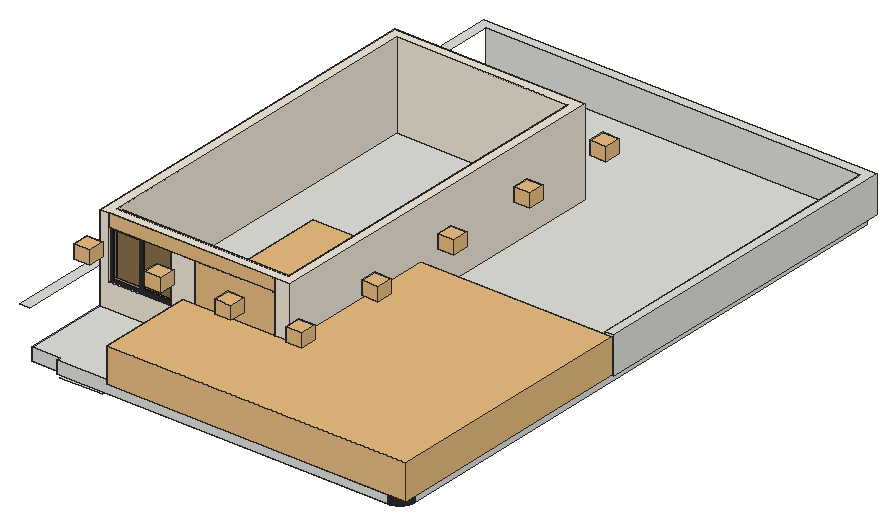
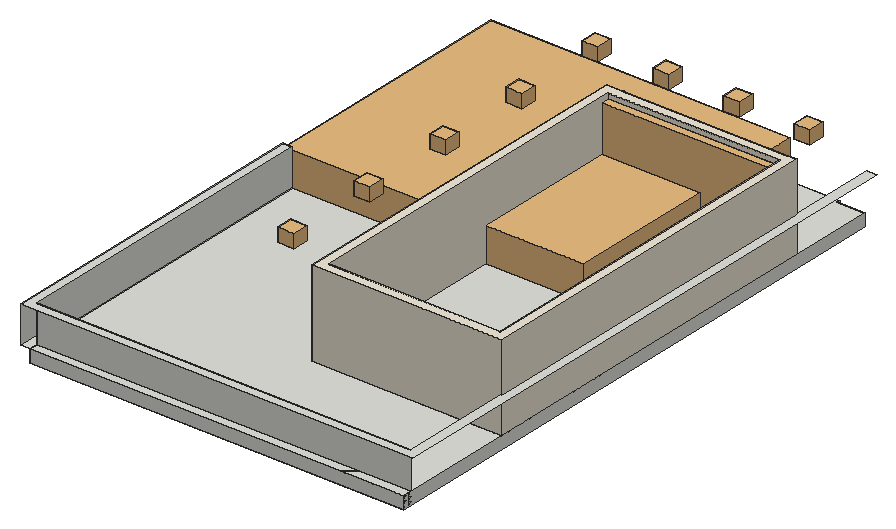
# SketchUp Ruby script. Lengths in inches.
U = 1.inch
M = Sketchup.active_model
def pt(a) = Geom::Point3d.new(a.map { |v| v * U })
def face(e, loops, mat)
  f = e.add_face(loops[0].map { |a| pt(a) })
  loops[1..].each { |l| e.add_face(l.map { |a| pt(a) }).erase! }
  f.material = f.back_material = mat if mat
  f
end
# faces: each face lists its corners as indices into pts; further lists are holes
def faces(e, pts, list, mat = nil) = list.each { |f| face(e, (f[0].is_a?(Array) ? f : [f]).map { |l| l.map { |i| pts[i] } }, mat) }
# xy, xz, yz: faces in a plane at the given z, y or x. An outline is a flat list of corners, or four numbers for a rectangle; further outlines are holes
def ring(l) = l.size == 4 ? [[l[0], l[1]], [l[2], l[1]], [l[2], l[3]], [l[0], l[3]]] : l.each_slice(2).to_a
def flat(e, list, mat, &to3) = list.each { |f| face(e, (f[0].is_a?(Array) ? f : [f]).map { |l| ring(l).map { |u, v| to3.(u, v) } }, mat) }
def xy(e, z, list, mat = nil) = flat(e, list, mat) { |x, y| [x, y, z] }
def xz(e, y, list, mat = nil) = flat(e, list, mat) { |x, z| [x, y, z] }
def yz(e, x, list, mat = nil) = flat(e, list, mat) { |y, z| [x, y, z] }
def lines(e, pts, list) = list.each { |a, b| e.add_line(pt(pts[a]), pt(pts[b])) }
# prism: a flat outline (further loops are holes) pulled along v
def prism(e, loops, v, mat = nil)
  f = face(e, loops, mat); d = Geom::Vector3d.new(v.map { |x| x * U })
  f.pushpull(f.normal.samedirection?(d) ? d.length : -d.length)
end
def box(e, o, s, mat = nil) = prism(e, [[o, [o[0] + s[0], o[1], o[2]], [o[0] + s[0], o[1] + s[1], o[2]], [o[0], o[1] + s[1], o[2]]]], [0, 0, s[2]], mat)
def at(x, y, z, deg = 0) = Geom::Transformation.translation(pt([x, y, z])) * Geom::Transformation.rotation(ORIGIN, Z_AXIS, deg.degrees)
def axes(o, x, y, z) = Geom::Transformation.new([*x, 0, *y, 0, *z, 0, *pt(o).to_a, 1])
def part(name) = M.definitions.add(name)
# library, detail: a bought-in or finely detailed component or shape, given as its bounding box
def library(name, o, s) = part(name).tap { |d| box(d.entities, o, s) }
def detail(e, o, s) = box(e.add_group.entities, o, s)
def put(e, d, t, mat = nil) = e.add_instance(d, t).tap { |i| i.material = mat if mat }
def group(e, t, mat = nil) = e.add_group.tap { |g| g.transformation = t; g.material = mat if mat }.entities
root = M.entities
M.materials.add("0027 AP L140 CRUSHED ICE").color = [241, 233, 217]
M.materials.add("Glass_Tinted_Gray").color = [0, 0, 0]
M.materials["Glass_Tinted_Gray"].alpha = 0.125
M.materials.add("[0135_DarkGray]").color = [81, 81, 81]
M.materials.add("[Metal Seamed]").color = [40, 40, 40]
M.materials.add("[Mirror 02]").color = [229, 229, 229]
M.materials.add("[Terrazzo Light Blue]").color = [196, 214, 227]
M.materials.add("[Wood Cherry Original]").color = [103, 58, 28]
M.materials.add("[Wood Fence]").color = [142, 67, 30]
c1 = library("Sliding glass door",[0,0,0],[5.83,106.3,82.68])
c2 = library("Group\#37",[0,0,0],[292,251.5,34])
c3 = library("Curtains",[0,0,0],[121.73,8.19,117.22])
c4 = library("Group\#52",[0,-0.5,0],[162,0.5,12])
c5 = part("PENTEK_RP Fineline 50S_Sliding_DoorCase_E1")
box(c5.entities,[0,0,0],[1.51,3.66,99.27],"[0135_DarkGray]")
c6 = part("PENTEK_RP Fineline 50S_SlidingDooe_Case_E2")
box(c6.entities,[0,0,0],[96.25,3.66,1.51],"[0135_DarkGray]")
c7 = part("pentek_RP Fineline 50S_SlidingDoor_Case")
put(c7.entities,c5,at(97.76,0,0))
put(c7.entities,c6,at(1.51,0,0))
put(c7.entities,c5,at(0,0,0))
put(c7.entities,c6,at(1.51,0,97.76))
c8 = part("PENTEK_RP Fineline 50S_SlidingDoor_GlazingBead_2")
box(c8.entities,[0,0,0],[0.56,0.59,94.39],"[0135_DarkGray]")
c9 = part("PENTEK_RP Fineline 50S_SlidingDoor_Glass")
box(c9.entities,[0,0,0],[46.58,0.16,94.39],"Glass_Tinted_Gray")
c10 = part("PENTEK_RP Fineline 50S_SlidingDoor_GlazingBead")
box(c10.entities,[0,0,0],[45.47,0.59,0.56],"[0135_DarkGray]")
c11 = part("PENTEK_RP Fineline 50S_SlidingDoor_Leaf_E1")
xy(c11.entities,0,[[0,0,0.93,1.97],[0.93,1.57,1.49,1.97]],"[0135_DarkGray]")
xy(c11.entities,96.25,[[0,0,0.93,0,0.93,1.57,1.49,1.57,1.49,1.97,0,1.97]],"[0135_DarkGray]")
xz(c11.entities,0,[[0,0,0.93,96.25]],"[0135_DarkGray]")
xz(c11.entities,1.57,[[0.93,0,1.49,95.32],[0.93,95.32,1.49,96.25]],"[0135_DarkGray]")
xz(c11.entities,1.97,[[0,0,1.49,96.25]],"[0135_DarkGray]")
yz(c11.entities,0,[[0,0,1.97,96.25]],"[0135_DarkGray]")
yz(c11.entities,0.93,[[0,0,1.57,0.93],[0,0.93,1.57,95.32],[0,95.32,1.57,96.25]],"[0135_DarkGray]")
yz(c11.entities,1.49,[[1.57,0,1.97,95.32],[1.57,95.32,1.97,96.25]],"[0135_DarkGray]")
c12 = part("PENTEK_RP Fineline 50S_SlidingDoor_Leaf_E2")
xy(c12.entities,0,[[0,0,0,1.57,0.56,1.57,0.56,1.97,46.02,1.97,46.02,1.57,46.58,1.57,46.58,0]],"[0135_DarkGray]")
xy(c12.entities,0.93,[[0,0,46.58,1.57]],"[0135_DarkGray]")
xy(c12.entities,1.49,[[0.56,1.57,46.02,1.97]],"[0135_DarkGray]")
xz(c12.entities,0,[[0,0,46.58,0.93]],"[0135_DarkGray]")
xz(c12.entities,1.57,[[0,0,0.56,0.93],[46.02,0,46.58,0.93],[0.56,0.93,46.02,1.49]],"[0135_DarkGray]")
xz(c12.entities,1.97,[[0.56,0,46.02,1.49]],"[0135_DarkGray]")
yz(c12.entities,0,[[0,0,1.57,0.93]],"[0135_DarkGray]")
yz(c12.entities,0.56,[[1.57,0,1.97,0.93],[1.57,0.93,1.97,1.49]],"[0135_DarkGray]")
yz(c12.entities,46.02,[[1.57,0,1.97,0.93],[1.57,0.93,1.97,1.49]],"[0135_DarkGray]")
yz(c12.entities,46.58,[[0,0,1.57,0.93]],"[0135_DarkGray]")
c13 = part("PENTEK_RP Fineline S_SlidingDoor_Leaf1")
put(c13.entities,c8,at(0.93,0,0.93))
put(c13.entities,c8,at(46.96,0,0.93))
put(c13.entities,c9,at(1.49,1.42,0.93))
put(c13.entities,c10,at(1.49,0,0.93))
put(c13.entities,c9,at(1.49,0.59,0.93),"[Terrazzo Light Blue]")
put(c13.entities,c11,at(0,0,0))
put(c13.entities,c11,axes([48.44,0,0],[-1,0,0],[0,1,0],[0,0,1]))
put(c13.entities,c12,axes([0.93,0,96.25],[1,0,0],[0,1,0],[0,0,-1]))
put(c13.entities,c12,at(0.93,0,0))
put(c13.entities,c10,at(1.49,0,94.77))
c14 = part("PENTEK_RP Fineline 50S_SlidingDoor_Leaf2")
put(c14.entities,c9,at(1.49,1.42,0.93))
put(c14.entities,c10,at(1.49,0,94.77))
put(c14.entities,c8,at(46.96,0,0.93))
put(c14.entities,c9,at(1.49,0.59,0.93),"[Mirror 02]")
put(c14.entities,c8,at(0.93,0,0.93))
put(c14.entities,c11,at(0,0,0))
put(c14.entities,c11,axes([48.44,0,0],[-1,0,0],[0,1,0],[0,0,1]))
put(c14.entities,c10,at(1.49,0,0.93))
put(c14.entities,c12,axes([0.93,0,96.25],[1,0,0],[0,1,0],[0,0,-1]))
put(c14.entities,c12,at(0.93,0,0))
c15 = part("PENTEK - Slimmest Steel Sliding Door / Window\#1")
put(c15.entities,c7,at(0,-1.88,-0.09))
put(c15.entities,c13,at(1.51,-2.27,1.42))
put(c15.entities,c14,at(49.32,-0.3,1.42))
c16 = library("3",[-5.94,-5.94,-13.08],[15.84,15.84,13.08])
xy(root,234,[[55.37,255,55.29,255.01,55.21,255.01,55.13,255.02,55.06,255.03,54.98,255.05,54.9,255.06,54.82,255.08,54.75,255.1,54.67,255.12,54.6,255.14,54.52,255.16,54.45,255.19,54.3,255.25,54.23,255.28,54.16,255.32,54.09,255.35,53.95,255.43,53.89,255.47,53.82,255.51,53.76,255.56,53.69,255.6,53.51,255.75,53.29,255.97,53.24,256.03,53.18,256.09,53.14,256.15,53.09,256.22,53.04,256.28,53,256.34,52.96,256.41,52.91,256.48,52.84,256.62,52.8,256.6875,52.77,256.76,52.68,256.97,52.65,257.05,52.61,257.2,52.59,257.28,52.57,257.35,52.55,257.43,52.54,257.51,52.53,257.58,52.51,257.74,52.51,257.82,52.5,257.9,52.5,258.13,52.51,258.21,52.51,258.29,52.52,258.37,52.53,258.44,52.55,258.52,52.56,258.6,52.58,258.68,52.6,258.75,52.62,258.83,52.64,258.9,52.66,258.98,52.69,259.05,52.75,259.2,52.78,259.27,52.82,259.34,52.85,259.41,52.93,259.55,52.97,259.61,53.01,259.68,53.06,259.74,53.1,259.81,53.25,259.99,53.47,260.21,53.53,260.26,53.59,260.32,53.65,260.36,53.72,260.41,53.78,260.46,53.84,260.5,53.91,260.54,53.98,260.59,54.12,260.66,54.1875,260.7,54.26,260.73,54.47,260.82,54.55,260.85,54.7,260.89,54.78,260.91,54.85,260.93,54.93,260.95,55.01,260.96,55.08,260.97,55.24,260.99,55.32,260.99,55.4,261,55.63,261,55.71,260.99,55.79,260.99,55.87,260.98,55.94,260.97,56.02,260.95,56.1,260.94,56.18,260.92,56.25,260.9,56.33,260.88,56.4,260.86,56.48,260.84,56.55,260.81,56.7,260.75,56.77,260.72,56.84,260.68,56.91,260.65,57.05,260.57,57.11,260.53,57.18,260.49,57.24,260.44,57.31,260.4,57.49,260.25,57.71,260.03,57.76,259.97,57.82,259.91,57.86,259.85,57.91,259.78,57.96,259.72,58,259.66,58.04,259.59,58.09,259.52,58.16,259.38,58.2,259.3125,58.23,259.24,58.32,259.03,58.35,258.95,58.39,258.8,58.41,258.72,58.43,258.65,58.45,258.57,58.46,258.49,58.47,258.42,58.49,258.26,58.49,258.18,58.5,258.1,58.5,257.87,58.49,257.79,58.49,257.71,58.48,257.63,58.47,257.56,58.45,257.48,58.44,257.4,58.42,257.32,58.4,257.25,58.38,257.17,58.36,257.1,58.34,257.02,58.31,256.95,58.25,256.8,58.22,256.73,58.18,256.66,58.15,256.59,58.07,256.45,58.03,256.39,57.99,256.32,57.94,256.26,57.9,256.19,57.75,256.01,57.53,255.79,57.47,255.74,57.41,255.68,57.35,255.64,57.28,255.59,57.22,255.54,57.16,255.5,57.09,255.46,57.02,255.41,56.88,255.34,56.8125,255.3,56.74,255.27,56.53,255.18,56.45,255.15,56.3,255.11,56.22,255.09,56.15,255.07,56.07,255.05,55.99,255.04,55.92,255.03,55.76,255.01,55.68,255.01,55.6,255]],"[Wood Fence]")
xy(root,252,[[51,210,93,210,93,213,99,213,99,214,368.95,214,369.1,214.01,369.29,214.04,369.48,214.0625,369.67,214.09,369.85,214.12,370.23,214.18,370.42,214.22,370.61,214.25,370.8,214.29,370.98,214.34,371.17,214.38,371.35,214.43,371.54,214.48,371.72,214.53,371.91,214.58,372.45,214.76,372.64,214.82,372.82,214.89,372.99,214.95,373.17,215.02,373.35,215.1,373.53,215.17,373.7,215.25,373.88,215.32,374.05,215.41,374.22,215.49,374.4,215.57,374.91,215.84,375.07,215.93,375.24,216.03,375.4,216.125,375.57,216.22,375.73,216.32,375.89,216.43,376.05,216.53,376.37,216.75,376.52,216.86,376.68,216.97,376.83,217.09,376.98,217.2,377.43,217.56,377.58,217.6875,377.72,217.8125,377.86,217.94,378.01,218.07,378.15,218.2,378.56,218.61,378.6875,218.74,378.82,218.88,378.95,219.02,379.08,219.17,379.2,219.31,379.33,219.46,379.45,219.6,379.81,220.05,379.92,220.21,380.04,220.36,380.15,220.52,380.26,220.67,380.36,220.83,380.47,220.99,380.57,221.15,380.68,221.31,380.78,221.48,380.87,221.64,380.97,221.81,381.0625,221.98,381.15,222.14,381.24,222.3125,381.33,222.48,381.42,222.66,381.58,223,381.66,223.18,381.74,223.35,381.88,223.71,381.95,223.88,382.02,224.0625,382.09,224.24,382.21,224.6,382.27,224.79,382.33,224.97,382.38,225.15,382.43,225.34,382.48,225.52,382.53,225.71,382.58,225.89,382.7,226.46,382.74,226.64,382.86,227.4,382.96,228.35,382.98,228.73,382.99,228.93,383,229.12,383,300,384,300,384,780,18,780,18,771,372,771,372,309,18,309,18,216.5,45,216.5,45,216,51,216]])
xy(root,264,[[384,459,384,771,18,771,18,780,393,780,393,459]])
xy(root,300,[[9,214,18,214,18,771,384,771,384,459,393,459,393,780,9,780]])
xz(root,260.99,[[55.24,231,55.32,234],[55.71,231,55.79,234]],"[Wood Fence]")
xz(root,261,[[55.4,231,55.47,234],[55.47,231,55.55,234],[55.55,231,55.63,234]],"[Wood Fence]")
xz(root,459,[[384,264,393,300]])
xz(root,771,[[18,264,384,300]])
yz(root,18,[[771,252,780,264]])
yz(root,52.5,[[257.9,231,257.97,234],[257.97,231,258.05,234],[258.05,231,258.13,234]],"[Wood Fence]")
yz(root,52.51,[[257.74,231,257.82,234],[258.21,231,258.29,234]],"[Wood Fence]")
yz(root,384,[[459,264,771,300]])
yz(root,393,[[459,264,780,300]])
p = [[53.57,255.7,231],[53.51,255.75,231],[53.51,255.75,234],[53.57,255.7,234],[53.45,255.81,231],[53.4,255.86,231],
  [53.4,255.86,234],[53.45,255.81,234],[53.34,255.92,231],[53.34,255.92,234],[53.29,255.97,231],[53.29,255.97,234],
  [53.24,256.03,231],[53.24,256.03,234],[53.18,256.09,231],[53.18,256.09,234],[53.14,256.15,231],[53.14,256.15,234],
  [53.09,256.22,231],[53.04,256.28,231],[53.04,256.28,234],[53.09,256.22,234],[53,256.34,231],[53,256.34,234],
  [52.96,256.41,231],[52.96,256.41,234],[52.91,256.48,231],[52.91,256.48,234],[52.875,256.55,231],[52.84,256.62,231],
  [52.84,256.62,234],[52.875,256.55,234],[52.8,256.6875,231],[52.8,256.6875,234],[52.77,256.76,231],[52.77,256.76,234],
  [52.74,256.83,231],[52.74,256.83,234],[52.71,256.9,231],[52.71,256.9,234],[52.68,256.97,231],[52.68,256.97,234],
  [52.65,257.05,231],[52.63,257.125,231],[52.63,257.125,234],[52.65,257.05,234],[52.61,257.2,231],[52.61,257.2,234],
  [52.59,257.28,231],[52.59,257.28,234],[52.57,257.35,231],[52.57,257.35,234],[52.55,257.43,231],[52.54,257.51,231],
  [52.54,257.51,234],[52.55,257.43,234],[52.53,257.58,231],[52.53,257.58,234],[52.52,257.66,231],[52.52,257.66,234],
  [52.51,257.74,231],[52.51,257.74,234],[52.51,257.82,231],[52.5,257.9,231],[52.5,257.9,234],[52.51,257.82,234],
  [52.5,258.13,231],[52.51,258.21,231],[52.51,258.21,234],[52.5,258.13,234],[52.51,258.29,231],[52.52,258.37,231],
  [52.52,258.37,234],[52.51,258.29,234],[52.53,258.44,231],[52.53,258.44,234],[52.55,258.52,231],[52.55,258.52,234],
  [52.56,258.6,231],[52.56,258.6,234],[52.58,258.68,231],[52.58,258.68,234],[52.6,258.75,231],[52.6,258.75,234],
  [52.62,258.83,231],[52.62,258.83,234],[52.64,258.9,231],[52.64,258.9,234],[52.66,258.98,231],[52.66,258.98,234],
  [52.69,259.05,231],[52.69,259.05,234],[52.72,259.125,231],[52.72,259.125,234],[52.75,259.2,231],[52.75,259.2,234],
  [52.78,259.27,231],[52.78,259.27,234],[52.82,259.34,231],[52.82,259.34,234],[52.85,259.41,231],[52.85,259.41,234],
  [52.89,259.48,231],[52.89,259.48,234],[52.93,259.55,231],[52.93,259.55,234],[52.97,259.61,231],[52.97,259.61,234],
  [53.01,259.68,231],[53.01,259.68,234],[53.06,259.74,231],[53.06,259.74,234],[53.1,259.81,231],[53.1,259.81,234],
  [53.15,259.87,231],[53.15,259.87,234],[53.2,259.93,231],[53.2,259.93,234],[53.25,259.99,231],[53.25,259.99,234],
  [53.31,260.05,231],[53.31,260.05,234],[53.36,260.1,231],[53.36,260.1,234],[53.42,260.16,231],[53.42,260.16,234],
  [53.47,260.21,231],[53.47,260.21,234],[53.53,260.26,231],[53.53,260.26,234],[53.59,260.32,231],[53.59,260.32,234],
  [53.65,260.36,231],[53.65,260.36,234],[53.72,260.41,231],[53.72,260.41,234],[53.78,260.46,231],[53.78,260.46,234],
  [53.84,260.5,231],[53.84,260.5,234],[53.91,260.54,231],[53.91,260.54,234],[53.98,260.59,231],[53.98,260.59,234],
  [57.05,260.57,231],[57.11,260.53,231],[57.11,260.53,234],[57.05,260.57,234],[54.05,260.625,231],[54.05,260.625,234],
  [54.12,260.66,231],[54.12,260.66,234],[56.84,260.68,231],[56.91,260.65,231],[56.91,260.65,234],[56.84,260.68,234],
  [56.98,260.61,231],[56.98,260.61,234],[54.1875,260.7,231],[54.1875,260.7,234],[54.26,260.73,231],[54.26,260.73,234],
  [54.33,260.76,231],[54.33,260.76,234],[56.7,260.75,231],[56.77,260.72,231],[56.77,260.72,234],[56.7,260.75,234],
  [54.4,260.79,231],[54.4,260.79,234],[54.47,260.82,231],[54.47,260.82,234],[54.55,260.85,231],[54.55,260.85,234],
  [54.625,260.87,231],[54.625,260.87,234],[56.4,260.86,231],[56.48,260.84,231],[56.48,260.84,234],[56.4,260.86,234],
  [56.55,260.81,231],[56.55,260.81,234],[56.625,260.78,231],[56.625,260.78,234],[54.7,260.89,231],[54.7,260.89,234],
  [54.78,260.91,231],[54.78,260.91,234],[54.85,260.93,231],[54.85,260.93,234],[54.93,260.95,231],[54.93,260.95,234],
  [55.01,260.96,231],[55.01,260.96,234],[56.02,260.95,231],[56.1,260.94,231],[56.1,260.94,234],[56.02,260.95,234],
  [56.18,260.92,231],[56.18,260.92,234],[56.25,260.9,231],[56.25,260.9,234],[56.33,260.88,231],[56.33,260.88,234],
  [55.08,260.97,231],[55.08,260.97,234],[55.16,260.98,231],[55.16,260.98,234],[55.24,260.99,231],[55.24,260.99,234],
  [55.32,260.99,231],[55.4,261,231],[55.4,261,234],[55.32,260.99,234],[55.63,261,231],[55.71,260.99,231],
  [55.71,260.99,234],[55.63,261,234],[55.79,260.99,231],[55.87,260.98,231],[55.87,260.98,234],[55.79,260.99,234],
  [55.94,260.97,231],[55.94,260.97,234]]
faces(root,p,[[0,1,2,3],[4,5,6,7],[1,4,7,2],[5,8,9,6],[8,10,11,9],[10,12,13,11],[12,14,15,13],[14,16,17,15],
  [18,19,20,21],[16,18,21,17],[19,22,23,20],[22,24,25,23],[24,26,27,25],[28,29,30,31],[26,28,31,27],[29,32,33,30],
  [32,34,35,33],[34,36,37,35],[36,38,39,37],[38,40,41,39],[42,43,44,45],[40,42,45,41],[43,46,47,44],[46,48,49,47],
  [48,50,51,49],[52,53,54,55],[50,52,55,51],[53,56,57,54],[56,58,59,57],[58,60,61,59],[62,63,64,65],[66,67,68,69],
  [70,71,72,73],[71,74,75,72],[74,76,77,75],[76,78,79,77],[78,80,81,79],[80,82,83,81],[82,84,85,83],[84,86,87,85],
  [86,88,89,87],[88,90,91,89],[90,92,93,91],[92,94,95,93],[94,96,97,95],[96,98,99,97],[98,100,101,99],[100,102,103,101],
  [102,104,105,103],[104,106,107,105],[106,108,109,107],[108,110,111,109],[110,112,113,111],[112,114,115,113],[114,116,117,115],[116,118,119,117],
  [118,120,121,119],[120,122,123,121],[122,124,125,123],[124,126,127,125],[126,128,129,127],[128,130,131,129],[130,132,133,131],[132,134,135,133],
  [134,136,137,135],[136,138,139,137],[138,140,141,139],[140,142,143,141],[144,145,146,147],[142,148,149,143],[148,150,151,149],[152,153,154,155],
  [153,156,157,154],[156,144,147,157],[150,158,159,151],[158,160,161,159],[160,162,163,161],[164,165,166,167],[165,152,155,166],[162,168,169,163],
  [168,170,171,169],[170,172,173,171],[172,174,175,173],[176,177,178,179],[177,180,181,178],[180,182,183,181],[182,164,167,183],[174,184,185,175],
  [184,186,187,185],[186,188,189,187],[188,190,191,189],[190,192,193,191],[194,195,196,197],[195,198,199,196],[198,200,201,199],[200,202,203,201],
  [202,176,179,203],[192,204,205,193],[204,206,207,205],[206,208,209,207],[210,211,212,213],[214,215,216,217],[218,219,220,221],[219,222,223,220],
  [222,194,197,223]],"[Wood Fence]")
g1 = group(root,at(18,216.5,252))
prism(g1,[[[366,563.5,0],[366,11.5,0],[366,11.3,0],[365.99,11.11,0],[365.99,10.91,0],[365.98,10.71,0],[365.97,10.52,0],[365.95,10.32,0],[365.9375,10.13,0],[365.92,9.93,0],[365.9,9.74,0],[365.87,9.54,0],[365.84,9.35,0],[365.82,9.15,0],[365.78,8.96,0],[365.75,8.77,0],[365.71,8.57,0],[365.67,8.38,0],[365.63,8.19,0],[365.59,8,0],[365.54,7.81,0],[365.49,7.62,0],[365.4375,7.43,0],[365.38,7.24,0],[365.33,7.05,0],[365.27,6.86,0],[365.2,6.68,0],[365.14,6.49,0],[365.07,6.31,0],[365,6.125,0],[364.93,5.94,0],[364.86,5.76,0],[364.78,5.58,0],[364.7,5.4,0],[364.62,5.22,0],[364.54,5.04,0],[364.45,4.87,0],[364.37,4.69,0],[364.27,4.52,0],[364.18,4.34,0],[364.09,4.17,0],[363.99,4,0],[363.89,3.83,0],[363.79,3.66,0],[363.6875,3.5,0],[363.58,3.33,0],[363.47,3.17,0],[363.36,3,0],[363.25,2.84,0],[363.14,2.68,0],[363.02,2.53,0],[362.9,2.37,0],[362.78,2.21,0],[362.66,2.06,0],[362.53,1.91,0],[362.41,1.76,0],[362.28,1.61,0],[362.15,1.46,0],[362.01,1.32,0],[361.88,1.17,0],[361.74,1.03,0],[361.61,0.89,0],[361.47,0.76,0],[361.33,0.62,0],[361.18,0.49,0],[361.04,0.35,0],[360.89,0.22,0],[360.74,0.09,0],[360.59,-0.03,0],[360.44,-0.16,0],[360.29,-0.28,0],[360.13,-0.4,0],[359.97,-0.52,0],[359.82,-0.64,0],[359.66,-0.75,0],[359.5,-0.86,0],[359.33,-0.97,0],[359.17,-1.08,0],[359,-1.1875,0],[358.84,-1.29,0],[358.67,-1.39,0],[358.5,-1.49,0],[358.33,-1.59,0],[358.16,-1.68,0],[357.98,-1.77,0],[357.81,-1.87,0],[357.63,-1.95,0],[357.46,-2.04,0],[357.28,-2.12,0],[357.1,-2.2,0],[356.92,-2.28,0],[356.74,-2.36,0],[356.56,-2.43,0],[356.375,-2.5,0],[356.19,-2.57,0],[356.01,-2.64,0],[355.82,-2.7,0],[355.64,-2.77,0],[355.45,-2.83,0],[355.26,-2.88,0],[355.07,-2.9375,0],[354.88,-2.99,0],[354.69,-3.04,0],[354.5,-3.09,0],[354.31,-3.13,0],[354.12,-3.17,0],[353.93,-3.21,0],[353.73,-3.25,0],[353.54,-3.28,0],[353.35,-3.32,0],[353.15,-3.34,0],[352.96,-3.37,0],[352.76,-3.4,0],[352.57,-3.42,0],[352.37,-3.4375,0],[352.18,-3.45,0],[351.98,-3.47,0],[351.79,-3.48,0],[351.59,-3.49,0],[351.39,-3.49,0],[351.2,-3.5,0],[351,-3.5,0],[27.5,-3.5,0],[27.5,0,0],[0,0,0],[0,563.5,0]]],[0,0,12])
put(root,c1,axes([189,300,264],[0,1,0],[-0.73378,0,0],[0,0,0.87087]))
put(root,c2,at(99,207.5,264),"[Metal Seamed]")
g2 = group(root,at(18,300,264),"0027 AP L140 CRUSHED ICE")
xy(g2,0,[[0,0,0,360,186,360,186,0,171,0,171,9,177,9,177,351,9,351,9,9,93,9,93,0]])
xy(g2,24,[[9,0,69,9]])
xy(g2,72,[[69,0,93,0.5],[9,0.5,69,9],[93,0.5,171,9]])
xy(g2,84,[[[0,0,9,0,9,0.5,171,0.5,171,0,186,0,186,360,0,360],[9,9,177,351]]])
xz(g2,0,[[0,0,93,0,93,72,69,72,69,24,9,24,9,84,0,84],[171,0,186,84]])
xz(g2,0.5,[[9,72,171,84]])
xz(g2,9,[[9,0,9,24,69,24,69,72,9,72,9,84,177,84,177,0,171,0,171,72,93,72,93,0]])
xz(g2,351,[[9,0,177,84]])
xz(g2,360,[[0,0,186,84]])
yz(g2,0,[[0,0,360,84]])
yz(g2,9,[[9,0,351,84],[0,24,9,72],[0,72,0.5,84]])
yz(g2,69,[[0,24,9,72]])
yz(g2,93,[[0,0,9,72]])
yz(g2,171,[[0,0,9,72],[0,72,0.5,84]])
yz(g2,177,[[9,0,351,84]])
yz(g2,186,[[0,0,360,84]])
put(g2,c3,axes([9,9,5.06],[1.38014,0,0],[0,1,0],[0,0,0.63062]))
put(g2,c4,at(9,0.5,72),"[Wood Cherry Original]")
put(root,c15,axes([27,302.77,288.04],[0.6044,0,0],[0,0.7182,0],[0,0,0.48352]))
put(root,c16,at(250.02,250.02,349.26))
put(root,c16,at(250.02,343.02,349.26))
put(root,c16,at(250.02,436.02,349.26))
put(root,c16,at(250.02,529.02,349.26))
put(root,c16,at(250.02,622.02,349.26))
put(root,c16,at(181.02,250.02,349.3))
put(root,c16,at(112.02,250.02,349.34))
put(root,c16,at(43.02,250.02,349.375))
